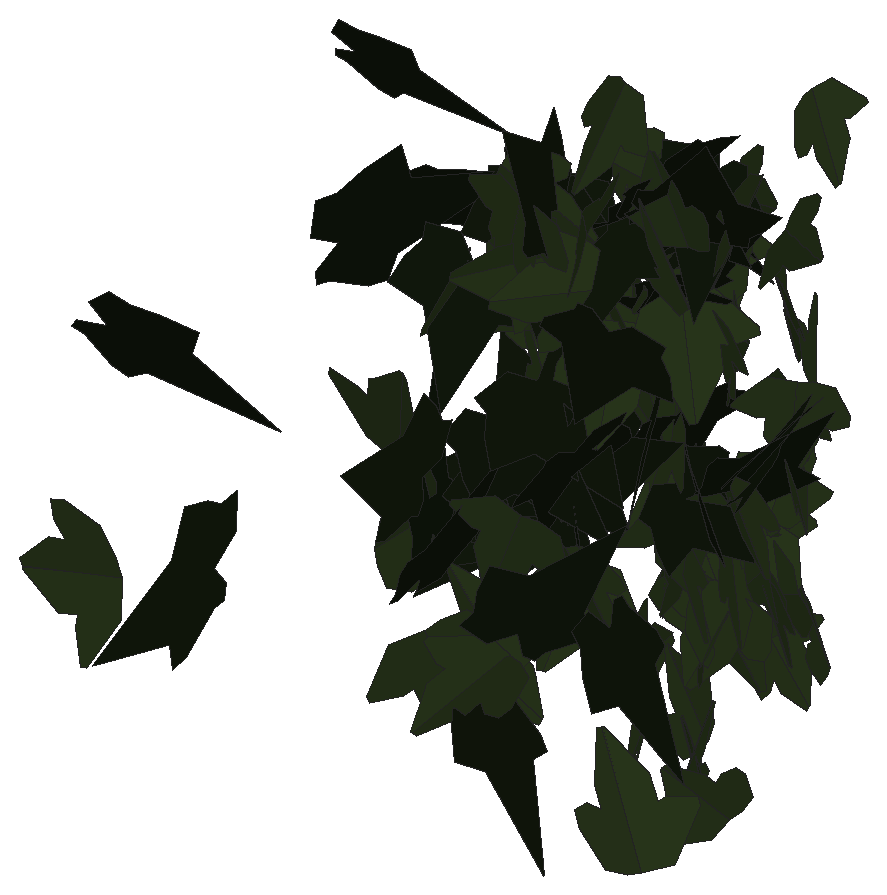
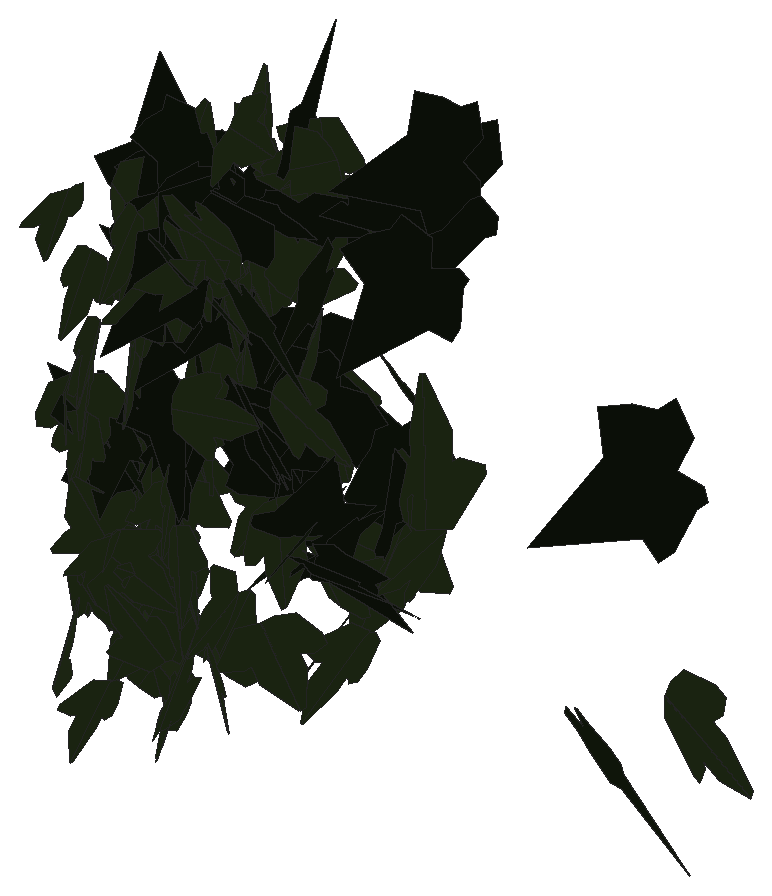
# SketchUp Ruby script. Lengths in inches.
U = 1.inch
M = Sketchup.active_model
def pt(a) = Geom::Point3d.new(a.map { |v| v * U })
def face(e, loops, mat)
  f = e.add_face(loops[0].map { |a| pt(a) })
  loops[1..].each { |l| e.add_face(l.map { |a| pt(a) }).erase! }
  f.material = f.back_material = mat if mat
  f
end
# faces: each face lists its corners as indices into pts; further lists are holes
def faces(e, pts, list, mat = nil) = list.each { |f| face(e, (f[0].is_a?(Array) ? f : [f]).map { |l| l.map { |i| pts[i] } }, mat) }
# xy, xz, yz: faces in a plane at the given z, y or x. An outline is a flat list of corners, or four numbers for a rectangle; further outlines are holes
def ring(l) = l.size == 4 ? [[l[0], l[1]], [l[2], l[1]], [l[2], l[3]], [l[0], l[3]]] : l.each_slice(2).to_a
def flat(e, list, mat, &to3) = list.each { |f| face(e, (f[0].is_a?(Array) ? f : [f]).map { |l| ring(l).map { |u, v| to3.(u, v) } }, mat) }
def xy(e, z, list, mat = nil) = flat(e, list, mat) { |x, y| [x, y, z] }
def xz(e, y, list, mat = nil) = flat(e, list, mat) { |x, z| [x, y, z] }
def yz(e, x, list, mat = nil) = flat(e, list, mat) { |y, z| [x, y, z] }
def lines(e, pts, list) = list.each { |a, b| e.add_line(pt(pts[a]), pt(pts[b])) }
# prism: a flat outline (further loops are holes) pulled along v
def prism(e, loops, v, mat = nil)
  f = face(e, loops, mat); d = Geom::Vector3d.new(v.map { |x| x * U })
  f.pushpull(f.normal.samedirection?(d) ? d.length : -d.length)
end
def box(e, o, s, mat = nil) = prism(e, [[o, [o[0] + s[0], o[1], o[2]], [o[0] + s[0], o[1] + s[1], o[2]], [o[0], o[1] + s[1], o[2]]]], [0, 0, s[2]], mat)
def at(x, y, z, deg = 0) = Geom::Transformation.translation(pt([x, y, z])) * Geom::Transformation.rotation(ORIGIN, Z_AXIS, deg.degrees)
def axes(o, x, y, z) = Geom::Transformation.new([*x, 0, *y, 0, *z, 0, *pt(o).to_a, 1])
def part(name) = M.definitions.add(name)
# library, detail: a bought-in or finely detailed component or shape, given as its bounding box
def library(name, o, s) = part(name).tap { |d| box(d.entities, o, s) }
def detail(e, o, s) = box(e.add_group.entities, o, s)
def put(e, d, t, mat = nil) = e.add_instance(d, t).tap { |i| i.material = mat if mat }
def group(e, t, mat = nil) = e.add_group.tap { |g| g.transformation = t; g.material = mat if mat }.entities
root = M.entities
M.materials.add("efeu1").color = [18, 25, 13]
M.materials.add("efeu2").color = [43, 57, 29]
c1 = part("ivyleaf_10")
p = [[0,0.5,-0.03],[-0.0625,2.02,-0.43],[-0.19,2.01,-0.46],[-0.54,1.05,-0.29],[-0.52,0.625,-0.18],[-0.83,0.76,-0.28],
  [-1.16,0.64,-0.33],[-1.15,0.33,-0.24],[-0.77,-0.39,0.02],[-0.3,-0.51,0.16],[0.04,-0.48,0.23],[-0.02,2.01,-0.4375],
  [-0.06,2.01,-0.43],[0.04,-0.49,0.23],[0.67,-0.49,0.14],[1.38,0.36,-0.2],[1.375,0.51,-0.24],[0.81,0.65,-0.19],
  [0.62,0.59,-0.15],[0.6,1.09,-0.28],[0.5,1.23,-0.31]]
faces(c1.entities,p,[[0,1,2,3,4,5,6,7,8,9,10],[11,12,0,13,14,15,16,17,18,19,20]],"efeu2")
c2 = part("ivyleaf_9")
p = [[1.54,2.16,1.25],[1.36,2.04,1.19],[-0.21,0.99,0.68],[-0.71,1.11,0.82],[-0.85,0.86,0.67],[-0.8,0.17,0.21],
  [-0.9,-0.01,0.1],[-0.67,-0.16,-0.02],[-0.08,-0.08,-0.05],[-0.03,-0.6,-0.4],[0.65,-0.88,-0.66],[0.83,-0.6,-0.49],
  [1.29,-0.42,-0.43],[1.8125,-0.07,-0.26],[1.21,0.44,0.15]]
faces(c2.entities,p,[[0,1,2,3,4,5,6,7,8,9,10,11,12,13,14]],"efeu1")
put(root,c1,axes([596.71,133.77,174.53],[-0.30615,-0.41951,0.59721],[-0.30119,-0.51728,-0.51776],[0.66478,-0.42756,0.04045]))
put(root,c2,axes([594.78,132.6,182.07],[0.34787,0.35599,0.95871],[0.71249,0.64209,-0.49695],[-0.73364,0.79238,-0.02802]))
put(root,c2,axes([596.23,133.9,181.48],[-0.19192,-0.79272,0.06221],[-0.00895,-0.06184,-0.8156],[0.79511,-0.19204,0.00583]))
put(root,c2,axes([595.73,133.22,177.87],[-0.51826,0.53164,0.3765],[-0.25808,0.27419,-0.74243],[-0.59816,-0.57893,-0.00588]))
put(root,c1,axes([597.46,133.53,177.39],[-0.71859,-0.22796,0.34437],[-0.33044,-0.0972,-0.75386],[0.24773,-0.7909,-0.00661]))
put(root,c1,axes([596.1,133.6875,181.25],[0.26846,-0.76288,0.01785],[0.00599,-0.01682,-0.80874],[0.76307,0.26853,0.00006]))
put(root,c2,axes([589.63,133.27,178.34],[1.00428,0.05327,0.3186],[0.31879,0.00457,-1.00562],[-0.05216,1.0536,-0.01175]))
put(root,c2,axes([595.67,133.44,176.02],[0.17338,0.84027,0.25704],[-0.09016,-0.2436,0.85715],[0.87407,-0.1918,0.03743]))
put(root,c2,axes([597.66,133.39,175.74],[-0.07709,-0.2401,0.78728],[0.77462,0.24615,0.15092],[-0.27825,0.75178,0.20203]))
put(root,c1,axes([595.81,133.52,174.69],[-0.53363,-0.67493,-0.35639],[0.29252,0.22081,-0.85615],[0.70497,-0.60251,0.08547]))
put(root,c1,axes([589.06,133.49,173.64],[0.35364,-0.23395,-0.96533],[-0.83665,0.48213,-0.42334],[0.53536,0.908,-0.02393]))
put(root,c2,axes([599.09,133.77,181.32],[0.41646,0.32888,-0.61181],[-0.46124,-0.40244,-0.5303],[-0.51936,0.62112,-0.01964]))
put(root,c1,axes([597.1,134.6,181.63],[-0.05158,-0.05444,-0.84053],[-0.42156,-0.72738,0.07298],[-0.72921,0.42435,0.01726]))
put(root,c2,axes([597.4,134.4,182.74],[-0.14889,0.32286,0.77607],[-0.26832,-0.76517,0.26685],[0.79657,-0.19739,0.23495]))
put(root,c1,axes([597.22,133.93,182.79],[-0.78719,0.03037,0.34186],[-0.34261,-0.01905,-0.78722],[-0.02025,-0.85801,0.02958]))
put(root,c1,axes([598.14,134.51,182.55],[0.03606,-0.52462,-0.62607],[0.18777,-0.60457,0.51742],[-0.79494,-0.1666,0.09382]))
put(root,c2,axes([598.99,134.01,175.8125],[0.47979,-0.68551,-0.32904],[-0.18178,0.27438,-0.8367],[0.73834,0.51301,0.00782]))
put(root,c2,axes([596.31,134.32,173.37],[0.41677,-0.82191,-0.03889],[-0.03403,0.02634,-0.92135],[0.82212,0.41775,-0.01843]))
put(root,c1,axes([597.625,134.86,181.125],[-0.11492,0.23357,0.79351],[-0.06998,-0.80101,0.22564],[0.82421,-0.03545,0.1298]))
put(root,c1,axes([596.47,134.43,174.42],[0.50285,0.01488,0.69028],[-0.69043,0.0057,0.50284],[0.00416,-0.854,0.01539]))
put(root,c1,axes([599.01,134.55,171.89],[0.81929,0.18705,0.36196],[-0.35276,-0.08108,0.84037],[0.20387,-0.89201,-0.00048]))
put(root,c2,axes([597.86,134.4375,178.46],[-0.11599,0.7771,-0.22786],[0.05811,-0.22161,-0.78535],[-0.80773,-0.12753,-0.02378]))
put(root,c1,axes([593.93,134.87,177.01],[-0.99537,0.16535,0.41323],[0.39223,-0.15257,1.00585],[0.21036,1.06688,0.0798]))
put(root,c1,axes([596.76,135.04,180.65],[-0.3993,-0.47547,-0.48066],[-0.31076,-0.3667,0.6209],[-0.60045,0.50597,-0.0017]))
put(root,c1,axes([596.65,134.69,182.9],[-0.36752,0.06462,-0.64624],[0.63554,-0.11715,-0.37315],[-0.13376,-0.73415,0.00266]))
put(root,c2,axes([596.25,134.64,178.36],[-0.05888,-0.17184,-0.88111],[0.65328,0.59743,-0.16017],[0.61572,-0.65031,0.08568]))
put(root,c2,axes([593.48,134.625,184.02],[0.79102,-0.14261,0.40968],[0.41323,-0.01149,-0.80187],[0.13198,0.89074,0.05524]))
put(root,c2,axes([597.04,134.64,179.3125],[-0.02867,-0.48102,-0.68461],[0.04949,0.68284,-0.48185],[0.83524,-0.05697,0.00505]))
put(root,c2,axes([594.91,134.6,176.09],[-0.02441,-0.46377,0.69519],[0.15817,0.68035,0.45943],[-0.82058,0.14494,0.06788]))
put(root,c2,axes([590.17,134.9375,173.46],[-0.91148,0.56442,0.00038],[-0.0004,0.00009,-1.07208],[-0.56442,-0.91148,0.00014]))
put(root,c2,axes([597.0625,135.5,176.28],[0.03761,-0.06093,0.8045],[0.13825,-0.79298,-0.06652],[0.79487,0.1408,-0.0265]))
put(root,c1,axes([594.34,134.38,175.71],[-0.00386,0.0414,0.85618],[-0.29824,0.80263,-0.04016],[-0.80362,-0.29807,0.01079]))
put(root,c2,axes([596.61,135.24,182.28],[-0.45957,-0.51143,-0.38377],[0.25365,0.28801,-0.68757],[0.58694,-0.52491,-0.00335]))
put(root,c2,axes([597.68,135.66,182.09],[-0.66137,-0.42226,-0.29014],[0.29571,0.07228,-0.77925],[0.41838,-0.71858,0.09211]))
put(root,c1,axes([599.32,135.125,181.67],[-0.41748,0.34946,-0.48835],[-0.3917,0.29235,0.54405],[0.45516,0.57211,0.02028]))
put(root,c1,axes([597.91,135.42,179.96],[0.5321,0.58455,-0.15723],[-0.10619,-0.11596,-0.79046],[-0.59594,0.54259,0.00046]))
put(root,c1,axes([597.28,135.34,175.86],[-0.59676,0.20671,-0.33164],[0.3083,-0.12294,-0.63141],[-0.24013,-0.67156,0.01351]))
put(root,c1,axes([597.51,135.62,180.58],[0.08323,0.67691,-0.4173],[-0.10248,-0.40695,-0.68056],[-0.78857,0.12433,0.0444]))
put(root,c2,axes([594.03,134.83,181.66],[0.62182,0.58303,0.19841],[0.09336,0.18945,-0.84932],[-0.60875,0.6246,0.07241]))
put(root,c1,axes([596.4375,135.4,178.77],[-0.50671,0.59166,-0.1416],[-0.09136,0.10819,0.77898],[0.60147,0.51488,-0.00098]))
put(root,c1,axes([598.97,135.66,182.34],[-0.70719,0.0268,-0.17998],[-0.1797,0.01065,0.70769],[0.02859,0.72965,-0.00372]))
put(root,c1,axes([599.51,135.98,171.99],[-0.31243,-0.36304,-0.47507],[-0.32746,-0.34459,0.47868],[-0.50027,0.45229,-0.01663]))
put(root,c1,axes([597.46,136.03,183.875],[0.067,0.52433,-0.54232],[-0.13177,-0.52795,-0.52671],[-0.74274,0.14096,0.04452]))
put(root,c1,axes([595.38,135.24,173.5625],[0.03723,0.63832,0.49842],[0.04781,0.49635,-0.63923],[-0.80845,0.05875,-0.01485]))
put(root,c2,axes([596.64,135.6,177.0625],[0.03264,0.00481,0.85548],[0.81331,-0.26569,-0.02953],[0.26533,0.81383,-0.01469]))
put(root,c2,axes([598.32,136.01,179.19],[-0.3918,0.17914,-0.64883],[0.59627,-0.25596,-0.43073],[-0.31231,-0.71342,-0.00838]))
put(root,c2,axes([595.27,136.27,176.03],[-0.11533,-0.76945,0.20891],[-0.01199,-0.20939,-0.77783],[0.79722,-0.11447,0.01852]))
put(root,c2,axes([598.91,136.08,182.28],[0.77575,0.16518,0.21654],[-0.21209,-0.04369,0.79313],[0.17085,-0.80421,0.00138]))
put(root,c1,axes([597.65,135.72,180.45],[-0.57125,0.34205,0.47985],[-0.42815,0.21828,-0.6653],[-0.4049,-0.7134,0.02651]))
put(root,c2,axes([595.15,136.41,175.98],[-0.79054,-0.15831,0.02287],[-0.02033,-0.01491,-0.80616],[0.15865,-0.79073,0.01062]))
put(root,c2,axes([597.67,135.64,182.03],[0.48505,0.57657,0.15317],[0.09544,0.11987,-0.75345],[-0.58888,0.49433,0.00405]))
put(root,c2,axes([598.61,135.6875,183.18],[0.20808,0.72287,0.17476],[0.04838,0.16793,-0.75222],[-0.74212,0.21363,-0.00003]))
put(root,c2,axes([595.4,136.57,175.82],[-0.7923,0.01174,0.15186],[-0.14986,-0.20395,-0.76608],[0.02724,-0.78051,0.20246]))
put(root,c1,axes([598.64,136.1875,180.4],[0.51609,0.64605,0.08333],[0.06619,0.05376,-0.82669],[-0.64804,0.52001,-0.01807]))
put(root,c1,axes([597.79,136.23,179.5],[-0.79672,-0.01289,-0.10164],[0.10227,-0.05234,-0.79502],[0.00614,-0.80147,0.05356]))
put(root,c2,axes([598.6,135.89,182.42],[0.58924,0.48535,0.05808],[0.0386,0.04448,-0.76333],[-0.48728,0.59043,0.00976]))
put(root,c1,axes([596.97,136.61,180.24],[-0.34201,0.14081,0.71519],[0.67441,-0.23862,0.36949],[0.27657,0.75599,-0.01658]))
put(root,c2,axes([595.37,136.17,181.65],[0.61014,-0.24442,-0.40215],[-0.35091,0.20244,-0.65545],[0.31357,0.70214,0.04899]))
put(root,c1,axes([597.68,136.43,173.04],[0.43634,-0.51091,-0.11973],[-0.06586,0.10116,-0.6717],[0.5206,0.44102,0.01537]))
put(root,c2,axes([597.22,136.1,177.77],[-0.07782,0.18492,0.73524],[-0.44157,0.58974,-0.19507],[-0.61627,-0.44591,0.04692]))
put(root,c2,axes([595.35,136.54,176.59],[0.45606,-0.66031,-0.13702],[-0.01081,0.15823,-0.79851],[0.67429,0.44914,0.07988]))
put(root,c1,axes([598.63,136.22,171.87],[0.30399,-0.53536,0.41652],[-0.20608,0.36196,0.61565],[-0.64624,-0.36726,-0.0004]))
put(root,c1,axes([598.42,136.47,176.69],[-0.41554,-0.64167,-0.0647],[0.04601,0.04728,-0.76437],[0.64329,-0.41788,0.01287]))
put(root,c2,axes([598.59,136.91,182.57],[-0.13211,-0.77907,-0.00625],[-0.00404,0.00702,-0.79017],[0.77908,-0.13207,-0.00516]))
put(root,c1,axes([597.79,135.97,173.89],[-0.05295,0.04542,0.7806],[-0.36301,0.69153,-0.06486],[-0.69255,-0.36595,-0.02568]))
put(root,c2,axes([597.875,136.1,180.52],[0.67856,0.45146,0.06735],[0.04072,0.06031,-0.81456],[-0.45464,0.67922,0.02756]))
put(root,c1,axes([598.04,136.55,178.15],[0.65318,-0.37356,-0.23313],[-0.14605,0.20965,-0.74515],[0.41541,0.66109,0.10458]))
put(root,c1,axes([598.05,137.02,175.38],[0.01319,-0.48023,-0.4668],[0.00289,-0.46685,0.48036],[-0.66971,-0.01148,-0.00712]))
put(root,c2,axes([595.58,136.61,176.5],[-0.57959,-0.51491,0.24337],[0.2056,0.13465,0.77452],[-0.53112,0.61402,0.03424]))
put(root,c1,axes([598.21,136.73,175.72],[-0.4443,0.35213,-0.33427],[0.23276,-0.24318,-0.56553],[-0.4261,-0.50001,0.03963]))
put(root,c2,axes([598.47,136.3,177.29],[0.28969,-0.30983,-0.64966],[-0.2747,0.5997,-0.4085],[0.66528,0.38254,0.11422]))
put(root,c1,axes([599.21,137.1,182.39],[0.24379,-0.59242,0.38429],[0.13048,-0.36175,-0.64046],[0.69399,0.27613,-0.01458]))
put(root,c1,axes([595.79,136.87,176.75],[-0.21551,-0.7639,-0.02712],[0.01158,0.02491,-0.7937],[0.76429,-0.21578,0.00438]))
put(root,c2,axes([598.125,136.54,180.37],[0.2346,0.7189,-0.07508],[0.01732,0.07332,0.75618],[0.7226,-0.23515,0.00625]))
put(root,c1,axes([595.62,136.75,179.14],[0.29505,-0.11662,-0.73562],[-0.68778,0.26101,-0.31724],[0.28585,0.74838,-0.00399]))
put(root,c2,axes([597.8,137.13,177.24],[0.14462,-0.00831,-0.76614],[0.76445,-0.05097,0.14486],[-0.05163,-0.77801,-0.00131]))
put(root,c2,axes([598.28,136.54,178.37],[0.12522,0.77737,-0.09638],[-0.01828,-0.09468,-0.78738],[-0.78311,0.12651,0.00297]))
put(root,c1,axes([596.93,137.0625,182.09],[-0.02803,-0.06275,-0.71995],[0.65712,-0.30207,0.00075],[-0.30077,-0.65412,0.06872]))
put(root,c1,axes([598.8,136.79,180.14],[-0.62622,0.371,0.08656],[-0.07414,0.04468,-0.72787],[-0.37368,-0.63059,-0.00065]))
put(root,c1,axes([595.92,137,174.35],[0.56629,0.49212,-0.25041],[-0.2857,-0.0458,-0.7361],[-0.4725,0.61749,0.14497]))
put(root,c1,axes([598.55,137.02,182.16],[-0.61333,-0.16436,0.25994],[-0.24083,-0.104,-0.63399],[0.19127,-0.65798,0.03527]))
put(root,c1,axes([599.06,137.04,177.03],[-0.6414,0.24795,-0.1796],[0.16068,-0.08226,-0.68742],[-0.26061,-0.66097,0.01818]))
put(root,c1,axes([598.43,137.57,180.68],[-0.05983,-0.06421,-0.74602],[-0.48682,-0.5653,0.08769],[-0.56893,0.49047,0.00341]))
put(root,c1,axes([598.09,137.08,172.3],[-0.40407,0.55374,-0.1092],[0.06529,-0.08754,-0.68549],[-0.56061,-0.40931,-0.00113]))
put(root,c1,axes([597.88,137.14,176.61],[-0.44068,-0.5992,-0.21261],[0.34162,-0.00498,-0.69406],[0.53623,-0.48926,0.26745]))
put(root,c1,axes([598.64,137.39,174.61],[-0.57892,-0.30647,0.36606],[-0.23095,-0.32377,-0.63632],[0.41783,-0.60359,0.15547]))
put(root,c2,axes([599.82,137.08,178.11],[-0.47183,0.62464,-0.04782],[0.02557,-0.04062,-0.7828],[-0.62595,-0.47251,0.00407]))
put(root,c2,axes([598.03,137.3,181.74],[-0.67679,0.36867,0.02666],[-0.05862,-0.05214,-0.76715],[-0.36496,-0.6753,0.07379]))
put(root,c1,axes([597.6,137.4375,175.74],[0.38477,-0.66296,0.06145],[0.0567,-0.03809,-0.76594],[0.66338,0.38778,0.02982]))
put(root,c2,axes([598.98,137.1,177.1],[0.45078,0.64029,-0.06184],[0.00848,0.06959,0.78236],[0.64321,-0.44965,0.03302]))
put(root,c1,axes([598.75,137.36,175.63],[-0.10835,0.66905,-0.14828],[0.02562,-0.14606,-0.67777],[-0.68481,-0.11133,-0.00189]))
put(root,c1,axes([597.5,137.42,182.1],[0.73198,-0.2266,-0.07968],[-0.07209,0.03653,-0.76613],[0.22913,0.7354,0.0135]))
put(root,c1,axes([597.96,137.16,176.86],[0.0714,-0.50795,-0.43559],[-0.04698,0.43317,-0.51284],[0.66749,0.08482,0.0105]))
put(root,c1,axes([597.83,137.5,172.31],[-0.23034,0.70236,0.12245],[0.0296,-0.11915,0.73912],[0.71234,0.23207,0.00888]))
put(root,c1,axes([597.875,137.1,174.72],[-0.10472,-0.35691,0.59645],[0.15257,0.57666,0.37186],[-0.67813,0.18486,-0.00844]))
put(root,c2,axes([596.13,137.07,178.62],[-0.18908,0.34056,0.67745],[-0.32202,0.59603,-0.38951],[-0.68646,-0.3734,-0.00388]))
put(root,c2,axes([596.12,137.43,181.45],[-0.57064,0.49708,0.06067],[-0.04983,0.03517,-0.75676],[-0.49829,-0.57278,0.00619]))
put(root,c1,axes([599.31,137.37,175.5625],[-0.44851,0.11191,0.53572],[-0.53255,0.07038,-0.46056],[-0.12612,-0.69513,0.03962]))
put(root,c1,axes([598.37,137.13,173.85],[0.26439,-0.10421,0.57448],[-0.3672,0.46062,0.25255],[-0.45393,-0.43331,0.13031]))
put(root,c1,axes([597.22,137.61,178.87],[-0.01409,0.02864,-0.69702],[-0.69707,0.02692,0.0152],[0.02752,0.69664,0.02807]))
put(root,c1,axes([599.29,137.52,175.23],[-0.54336,0.4269,-0.01992],[0.01818,-0.00911,-0.69099],[-0.42698,-0.54365,-0.00406]))
put(root,c1,axes([598.18,137.57,180.92],[0.17494,0.70188,0.01688],[0.00086,0.01718,-0.72334],[-0.70208,0.17491,0.00332]))
put(root,c1,axes([597.22,137.53,181.65],[0.43044,0.61919,0.13479],[0.07308,0.11336,-0.75409],[-0.62946,0.43658,0.00463]))
put(root,c1,axes([598.3,137.21,174.68],[-0.0238,0.49786,0.49867],[-0.08136,0.49367,-0.49676],[-0.69994,-0.07431,0.04078]))
put(root,c2,axes([597.64,137.41,181.63],[0.74766,0.16727,-0.0198],[-0.0199,-0.00173,-0.76614],[-0.16726,0.74792,0.00265]))
put(root,c1,axes([598.21,137.7,174.35],[-0.70691,-0.0504,-0.23627],[0.23612,0.01034,-0.70867],[0.05108,-0.74527,0.00614]))
put(root,c2,axes([599.44,137.34,177.92],[-0.00481,0.73457,0.24139],[-0.08885,0.23927,-0.72989],[-0.76809,-0.03228,0.08292]))
put(root,c1,axes([598.75,138.04,175.65],[0.41383,0.34265,-0.39183],[-0.302,-0.24965,-0.53728],[-0.42395,0.51231,0.00025]))
put(root,c1,axes([598.6,138.17,175.53],[-0.29074,-0.34286,0.56571],[-0.37444,-0.42411,-0.44949],[0.54532,-0.47402,-0.00702]))
put(root,c1,axes([599.53,137.92,178.53],[-0.60907,-0.40011,0.07551],[-0.02511,-0.0987,-0.72552],[0.4064,-0.60575,0.06834]))
put(root,c1,axes([598.66,137.49,179.52],[0.21535,-0.37261,-0.62387],[-0.16907,0.60714,-0.42098],[0.70673,0.25878,0.08939]))
put(root,c1,axes([598.67,137.52,182.04],[0.00291,-0.44298,-0.59748],[0.03988,0.59672,-0.44222],[0.74271,-0.03031,0.02609]))
put(root,c1,axes([599.39,138,174.96],[-0.29668,0.03985,0.59004],[-0.58527,0.07487,-0.29934],[-0.0848,-0.65617,0.00168]))
put(root,c1,axes([599.39,137.97,177.42],[-0.34182,0.60905,0.1312],[-0.11415,0.08589,-0.69612],[-0.61247,-0.35592,0.05651]))
put(root,c1,axes([598.67,138.28,175.81],[0.10141,0.63143,0.01278],[-0.00164,0.01321,-0.63951],[-0.63156,0.10135,0.00371]))
put(root,c1,axes([599.26,138.09,181.32],[-0.06572,-0.50292,-0.45112],[0.05931,0.4472,-0.50719],[0.67299,-0.08852,0.00065]))
put(root,c1,axes([598.95,138.34,180.1],[-0.46741,0.42153,0.17021],[-0.11978,0.1213,-0.62934],[-0.43853,-0.48242,-0.00952]))
put(root,c1,axes([596.85,138.41,176.53],[0.13707,-0.62621,-0.30183],[-0.07743,0.29198,-0.64093],[0.69083,0.15698,-0.01195]))
put(root,c1,axes([599.09,138.45,178.16],[-0.60111,0.18282,0.11682],[-0.10992,0.04004,-0.62827],[-0.18704,-0.61105,-0.00621]))
put(root,c1,axes([599,138.44,179.54],[-0.44443,0.30795,0.35546],[-0.28684,0.21008,-0.54064],[-0.3727,-0.5289,-0.00778]))
put(root,c1,axes([598.71,138.37,176.26],[0.32499,0.52898,-0.35342],[0.19491,0.29499,0.62075],[0.60558,-0.37882,-0.01013]))
put(root,c1,axes([599.48,138.35,178.78],[-0.13022,0.29519,-0.60342],[-0.21608,0.56358,0.32233],[0.63605,0.25189,-0.01404]))
put(root,c1,axes([597.2,138.79,174.47],[0.51539,-0.01901,-0.45169],[0.45007,-0.04296,0.51536],[-0.04259,-0.68396,-0.01982]))
put(root,c1,axes([599.15,138.96,173.41],[-0.43134,0.5179,0.06245],[0.03632,-0.05102,0.67398],[0.52039,0.43284,0.00473]))
put(root,c1,axes([599.14,138.97,183.12],[0.06132,0.63722,0.08643],[0.02011,0.08488,-0.64006],[-0.64274,0.06345,-0.01178]))
put(root,c1,axes([598.22,139,173.22],[0.03494,0.61428,0.27477],[0.00163,0.27506,-0.61514],[-0.67293,0.03256,0.01278]))
